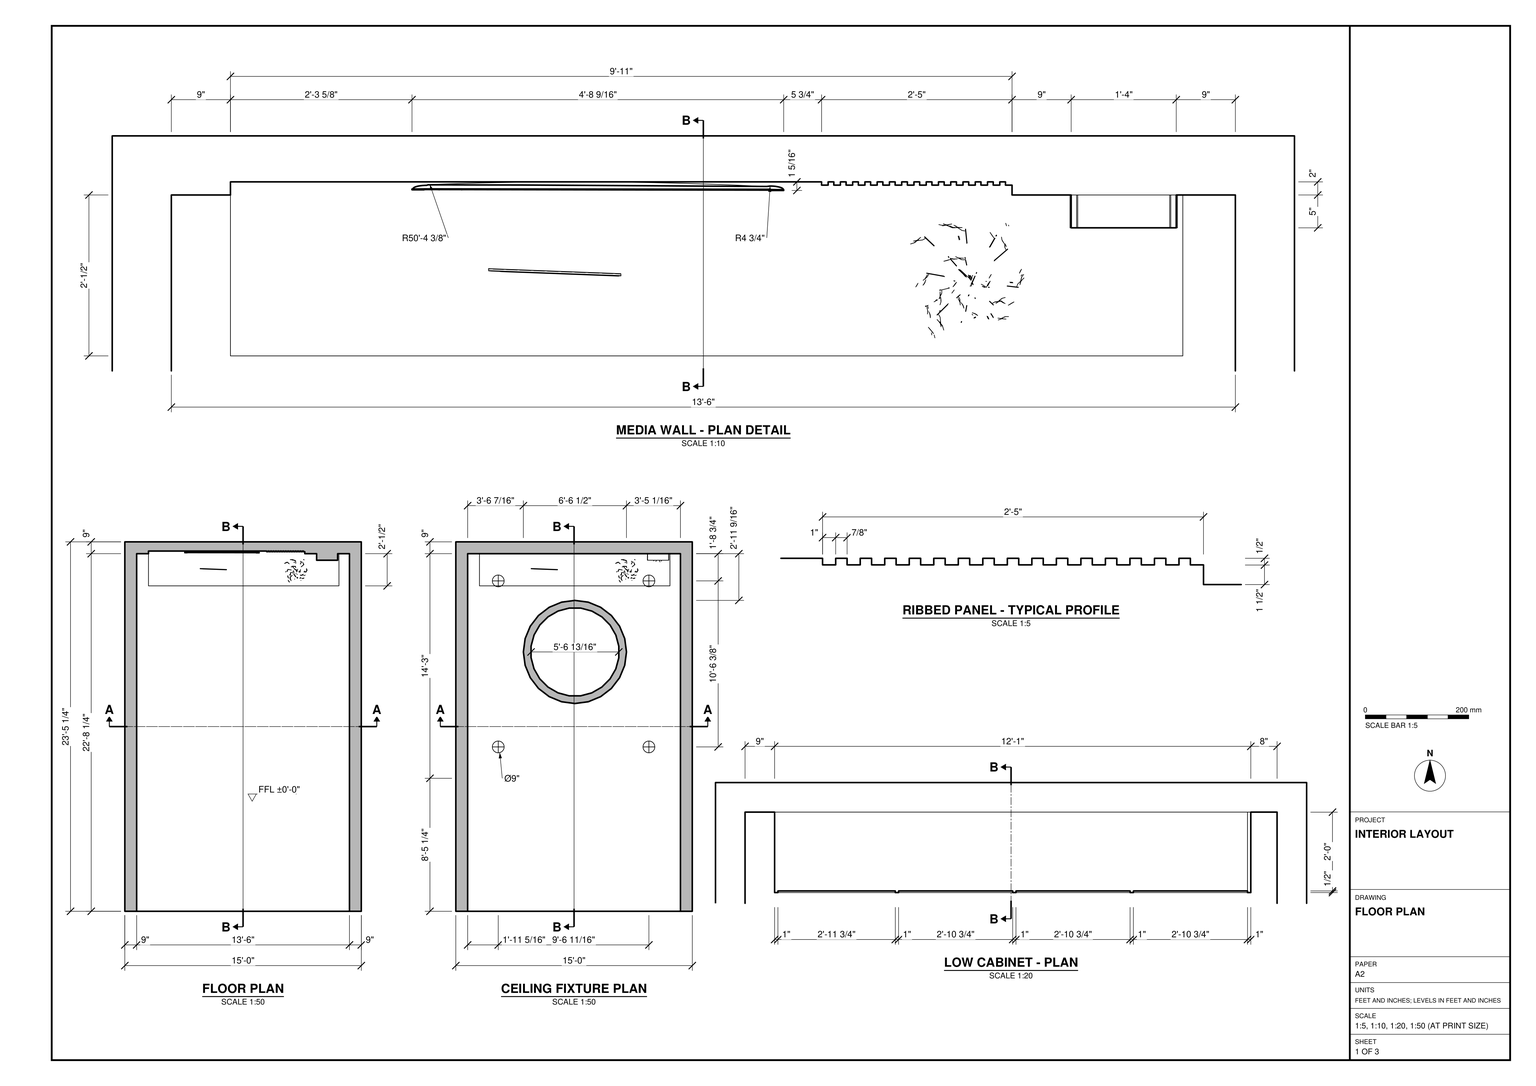
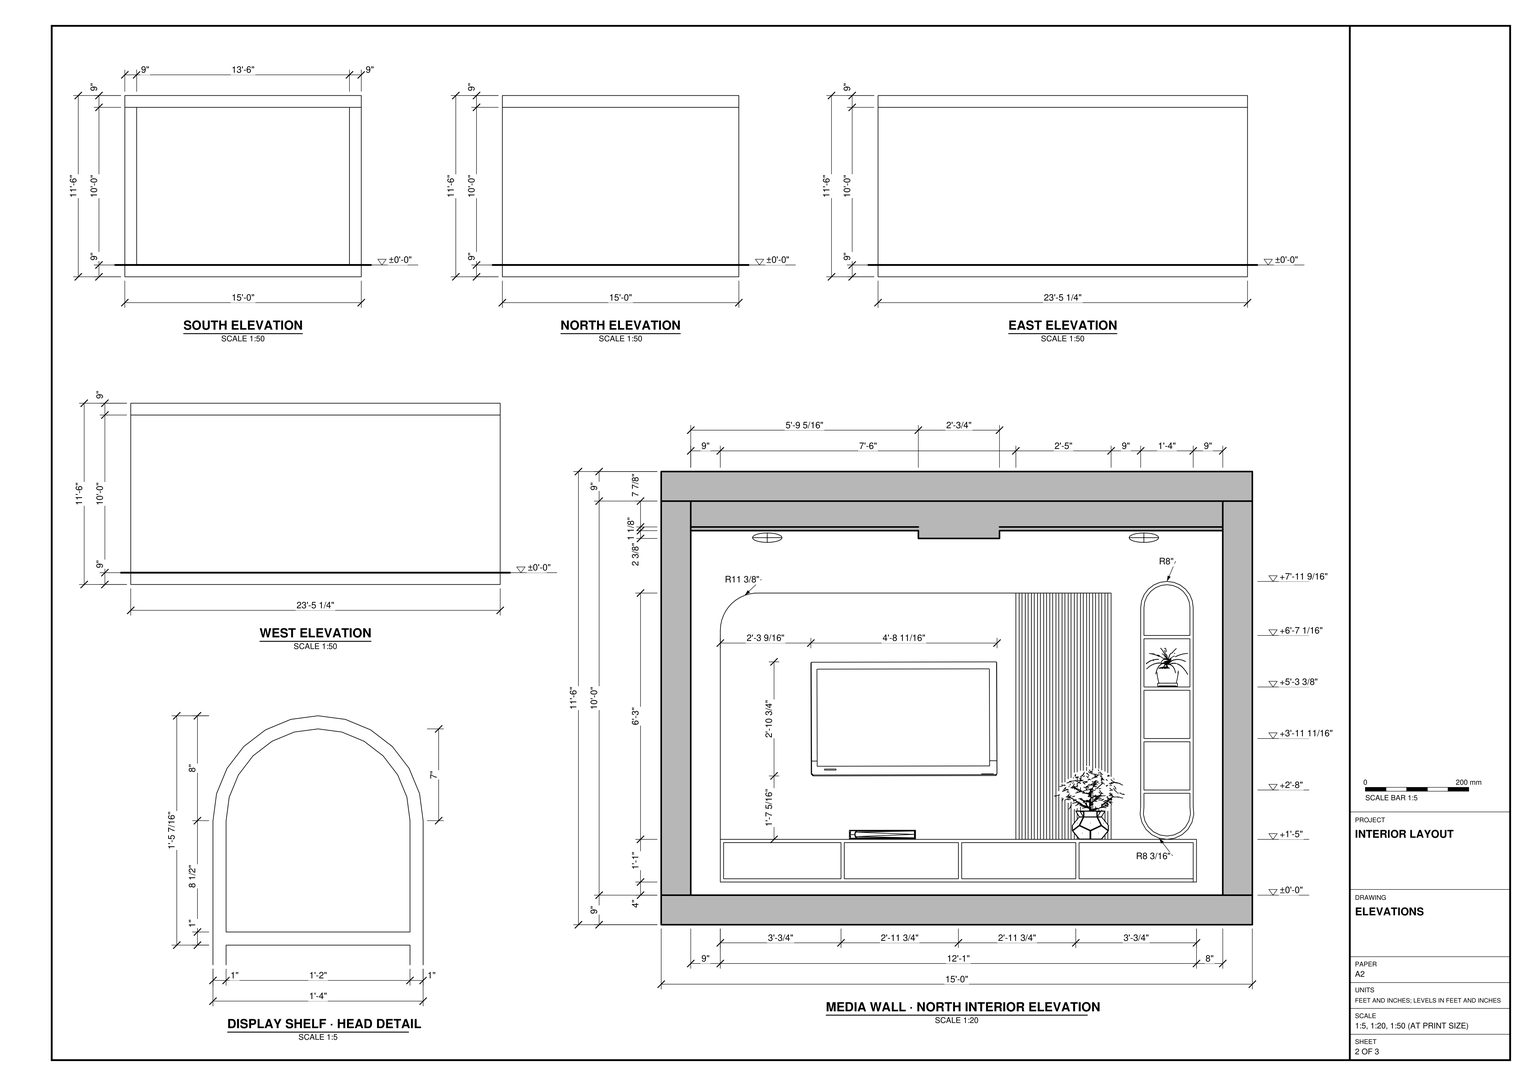
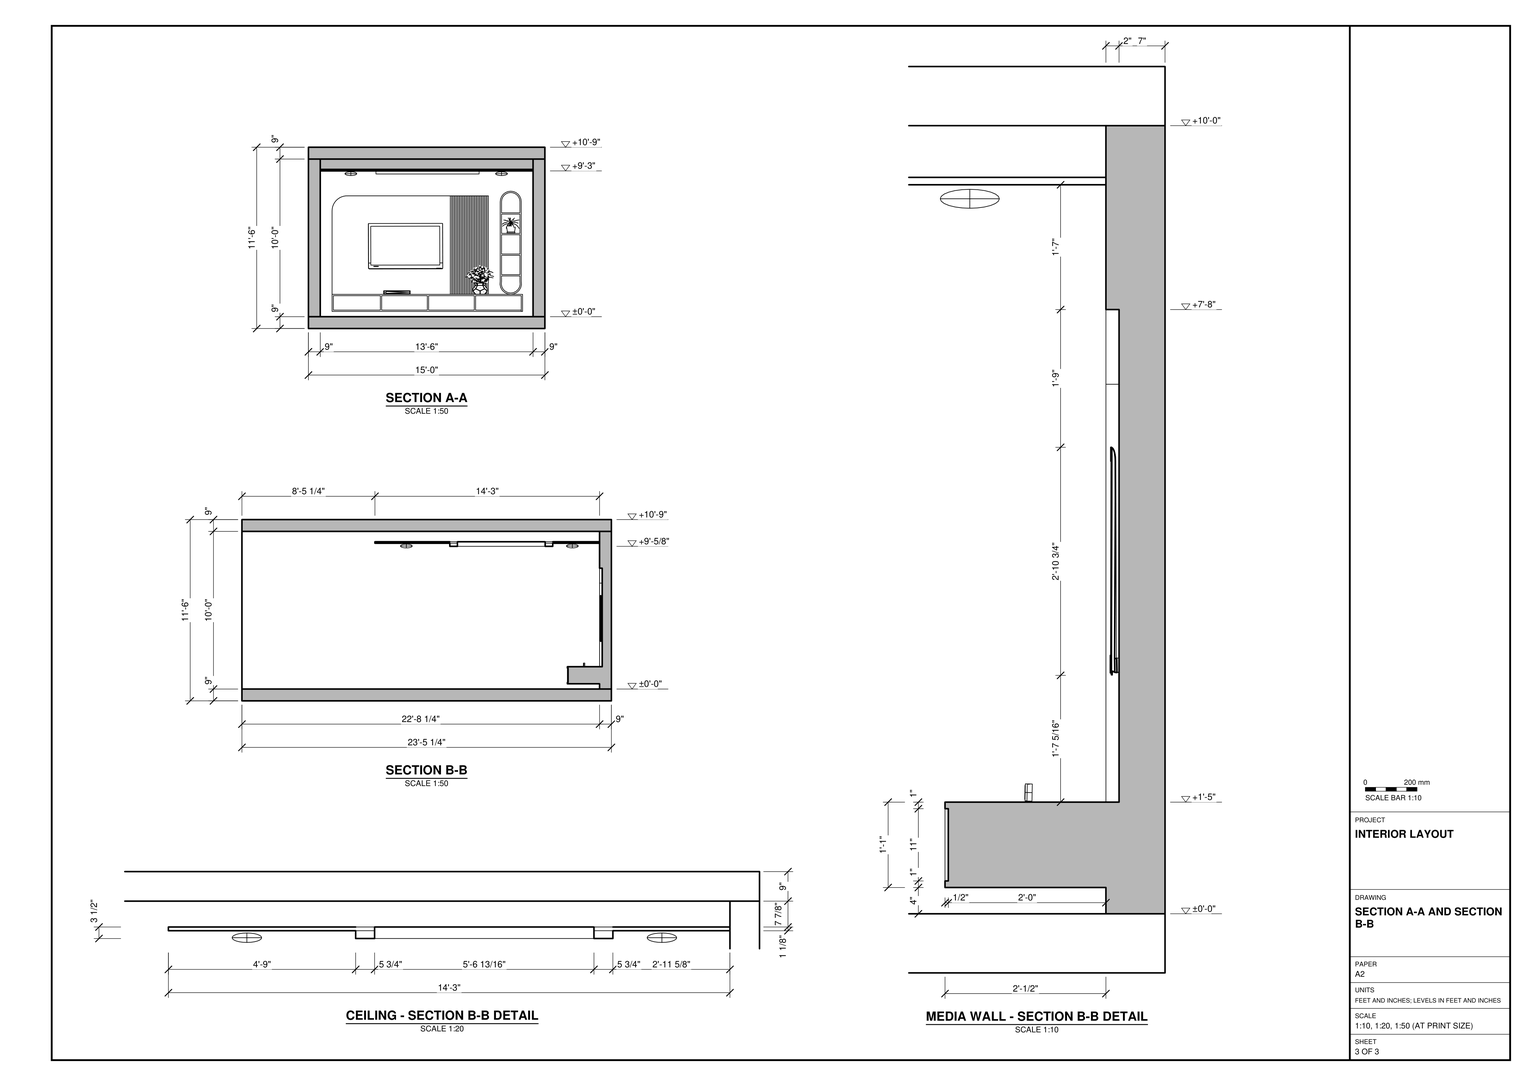
Build the media room in SketchUp from task_files/diagram_01.pdf. Work in feet and inches. Set the finished floor at ±0'-0" and make the shell 15'-0" wide, 23'-5 1/4" long and 11'-6" high overall. Model the north wall and both side walls at 9" thick, leaving the south end open as shown in plan. Use 9" floor and roof slabs with 10'-0" clear between them.

Use the north interior elevation to lay out the media wall. Float the low cabinet above the floor and divide its front into four bays. Mount the television on the smooth panel with the rounded upper left corner. Form the vertical ribs to its right using the profile detail, then add the narrow open display shelf with rounded ends. Place the small media device and potted plants where shown. Use the ceiling plan and section B-B to position the lowered ceiling panel, central ring fixture and smaller ceiling lights.

Decor and loose items may be any suitable library components. Keep the walls, slabs, ceiling panel and each furniture or joinery piece in separate groups or components, and use components for repeated parts. Save one SketchUp model as output_files/media_room_with_built_in_cabinetry_and_ceiling_fixtures.skp.

# SketchUp Ruby script. Lengths in inches.
U = 1.inch
M = Sketchup.active_model
def pt(a) = Geom::Point3d.new(a.map { |v| v * U })
def face(e, loops, mat)
  f = e.add_face(loops[0].map { |a| pt(a) })
  loops[1..].each { |l| e.add_face(l.map { |a| pt(a) }).erase! }
  f.material = f.back_material = mat if mat
  f
end
# faces: each face lists its corners as indices into pts; further lists are holes
def faces(e, pts, list, mat = nil) = list.each { |f| face(e, (f[0].is_a?(Array) ? f : [f]).map { |l| l.map { |i| pts[i] } }, mat) }
# xy, xz, yz: faces in a plane at the given z, y or x. An outline is a flat list of corners, or four numbers for a rectangle; further outlines are holes
def ring(l) = l.size == 4 ? [[l[0], l[1]], [l[2], l[1]], [l[2], l[3]], [l[0], l[3]]] : l.each_slice(2).to_a
def flat(e, list, mat, &to3) = list.each { |f| face(e, (f[0].is_a?(Array) ? f : [f]).map { |l| ring(l).map { |u, v| to3.(u, v) } }, mat) }
def xy(e, z, list, mat = nil) = flat(e, list, mat) { |x, y| [x, y, z] }
def xz(e, y, list, mat = nil) = flat(e, list, mat) { |x, z| [x, y, z] }
def yz(e, x, list, mat = nil) = flat(e, list, mat) { |y, z| [x, y, z] }
def lines(e, pts, list) = list.each { |a, b| e.add_line(pt(pts[a]), pt(pts[b])) }
# prism: a flat outline (further loops are holes) pulled along v
def prism(e, loops, v, mat = nil)
  f = face(e, loops, mat); d = Geom::Vector3d.new(v.map { |x| x * U })
  f.pushpull(f.normal.samedirection?(d) ? d.length : -d.length)
end
def box(e, o, s, mat = nil) = prism(e, [[o, [o[0] + s[0], o[1], o[2]], [o[0] + s[0], o[1] + s[1], o[2]], [o[0], o[1] + s[1], o[2]]]], [0, 0, s[2]], mat)
def at(x, y, z, deg = 0) = Geom::Transformation.translation(pt([x, y, z])) * Geom::Transformation.rotation(ORIGIN, Z_AXIS, deg.degrees)
def axes(o, x, y, z) = Geom::Transformation.new([*x, 0, *y, 0, *z, 0, *pt(o).to_a, 1])
def part(name) = M.definitions.add(name)
# library, detail: a bought-in or finely detailed component or shape, given as its bounding box
def library(name, o, s) = part(name).tap { |d| box(d.entities, o, s) }
def detail(e, o, s) = box(e.add_group.entities, o, s)
def put(e, d, t, mat = nil) = e.add_instance(d, t).tap { |i| i.material = mat if mat }
def group(e, t, mat = nil) = e.add_group.tap { |g| g.transformation = t; g.material = mat if mat }.entities
root = M.entities
M.materials.add("Emissive").color = [239, 214, 214]
M.materials.add("[0014_DarkSalmon]").color = [235, 180, 161]
M.materials.add("[0024_OrangeRed]").color = [254, 124, 76]
M.materials.add("[0134_DimGray]").color = [105, 105, 105]
M.materials.add("[0136_Charcoal]").color = [35, 35, 35]
M.materials.add("[0137_Black]").color = [0, 0, 0]
M.materials.add("[Carrera Marble]").color = [207, 207, 207]
c1 = library("Flat panel television",[-0.83,-0.0625,-0.19],[1.35,37.19,23.93])
c2 = part("skpA6C3")
xy(c2.entities,2.36,[[-169.4375,74.49,-169.56,74.75,-167.28,75.78,-167.16,75.52]])
xy(c2.entities,2.39,[[-169.39,74.48,-167.18,75.48,-169.18,74.58],[-169.39,74.48,-167.1875,75.5,-169.39,74.5],[-169.39,74.48,-169.18,74.58,-167.1875,75.5],[-169.18,74.58,-167.18,75.48,-167.1875,75.5]])
xy(c2.entities,2.8,[[-169.39,74.49,-169.39,74.5,-167.1875,75.5,-167.18,75.49,-169.18,74.58]])
xy(c2.entities,2.83,[[-169.4375,74.49,-167.16,75.52,-167.28,75.78,-169.56,74.75]])
xz(c2.entities,74.49,[[-169.4375,2.59,-169.39,2.8,-169.4375,2.83]])
yz(c2.entities,-169.39,[[74.48,2.39,74.5,2.39,74.48,2.6],[74.5,2.39,74.5,2.6,74.48,2.6],[74.48,2.6,74.5,2.6,74.5,2.8],[74.48,2.6,74.5,2.8,74.49,2.8]])
yz(c2.entities,-167.18,[[75.48,2.39,75.44,2.6,75.4375,2.41],[75.48,2.39,75.49,2.6,75.44,2.79,75.44,2.6],[75.49,2.6,75.49,2.8,75.44,2.79]])
p = [[-167.18,75.48,2.39],[-169.39,74.48,2.39],[-167.16,75.52,2.36],[-169.4375,74.49,2.36],[-167.1875,75.5,2.39],[-167.1875,75.5,2.6],
  [-167.1875,75.5,2.8],[-169.39,74.5,2.8],[-169.39,74.5,2.6],[-169.39,74.5,2.39],[-169.4375,74.49,2.59],[-169.39,74.48,2.6],
  [-169.18,74.58,2.39],[-167.18,75.4375,2.41],[-169.15,74.55,2.41],[-167.18,75.44,2.6],[-169.19,74.52,2.48],[-169.23,74.56,2.46],
  [-169.56,74.75,2.36],[-169.56,74.75,2.59],[-167.28,75.78,2.59],[-167.28,75.78,2.36],[-167.16,75.52,2.59],[-167.18,75.49,2.6],
  [-169.22,74.52,2.6],[-169.25,74.55,2.6],[-169.19,74.53,2.73],[-169.39,74.49,2.8],[-169.23,74.56,2.73],[-167.18,75.44,2.79],
  [-169.56,74.75,2.83],[-167.28,75.78,2.83],[-167.16,75.52,2.83],[-167.18,75.49,2.8],[-169.15,74.55,2.79],[-169.18,74.58,2.8],
  [-169.4375,74.49,2.83]]
faces(c2.entities,p,[[0,1,2],[1,3,2],[4,5,6,7,8,9],[10,3,1],[11,10,1],[12,0,13,14],[15,16,13],[16,14,13],
  [17,12,14],[16,17,14],[18,19,20,21],[2,21,20,22],[22,23,0],[22,0,2],[4,0,23],[5,4,23],
  [24,25,16],[25,17,16],[16,15,26,24],[27,10,11],[28,25,24],[29,26,15],[28,24,26],[19,30,31,20],
  [22,20,31,32],[22,33,23],[32,33,22],[5,23,33],[6,5,33],[29,34,26],[35,28,26],[35,26,34],
  [32,36,33],[27,35,33,36],[35,34,29,33]])
c3 = part("speaker")
put(c3.entities,c2,axes([-348.49,31.79,126.79],[0,-0.40035,0.91636],[0,0.91636,0.40035],[-1,0,0]))
c4 = library("4",[-16.3,-15.81,0],[32.6,31.62,37.8])
c5 = library("granite type garden pot + desert rose wine plant",[-22.7,-22.54,0],[44.26,46.62,61.81])
c6 = part("Group35\#1")
p = [[0,0,0],[0,0,-0.26],[-0.06,0,-0.26],[0.39,-0.44,0],[-0.39,-0.44,0],[0.39,0.44,0],
  [0.39,0,0],[-0.39,0.44,0],[0.06,0,-0.26],[-0.39,0,0],[0,0,-0.42]]
lines(c6.entities,p,[[0,1],[1,2],[3,4],[5,6],[7,5],[1,8],[9,0],[0,6],[8,10],[4,9],[6,3],[2,10],
  [9,7]])
c7 = part("Rectangle Light")
put(c7.entities,c6,at(0,0,0))
c8 = library("Sphere Light",[-4.5,-4.5,-4.5],[9,9,9])
xy(root,-9,[[0,0,180,281.25]])
xy(root,0,[[0,0,9,0,9,272.25,171,272.25,171,0,180,0,180,281.25,0,281.25],[9,0,171,272.25]])
xy(root,4,[[18,247.75,162,272.25],[162,247.75,163,272.25]])
xy(root,5,[[19,247.75,54.75,248.25],[55.75,247.75,90.5,248.25],[91.5,247.75,126.25,248.25],[127.25,247.75,162,248.25]])
xy(root,16,[[19,247.75,54.75,248.25],[55.75,247.75,90.5,248.25],[91.5,247.75,126.25,248.25],[127.25,247.75,162,248.25]])
xy(root,17,[[18,247.75,163,247.75,163,272.25,137,272.25,137,273.75,136,273.75,136,274.25,135.13,274.25,135.13,273.75,134.13,273.75,134.13,274.25,133.27,274.25,133.27,273.75,132.27,273.75,132.27,274.25,131.4,274.25,131.4,273.75,130.4,273.75,130.4,274.25,129.53,274.25,129.53,273.75,128.53,273.75,128.53,274.25,127.67,274.25,127.67,273.75,126.67,273.75,126.67,274.25,125.8,274.25,125.8,273.75,124.8,273.75,124.8,274.25,123.93,274.25,123.93,273.75,122.93,273.75,122.93,274.25,122.07,274.25,122.07,273.75,121.07,273.75,121.07,274.25,120.2,274.25,120.2,273.75,119.2,273.75,119.2,274.25,118.33,274.25,118.33,273.75,117.33,273.75,117.33,274.25,116.47,274.25,116.47,273.75,115.47,273.75,115.47,274.25,114.6,274.25,114.6,273.75,113.6,273.75,113.6,274.25,112.73,274.25,112.73,273.75,111.73,273.75,111.73,274.25,110.87,274.25,110.87,273.75,109.87,273.75,109.87,274.25,109,274.25,109,273.75,108,273.75,108,274.25,18,274.25]],"[Carrera Marble]")
xy(root,31.02,[[147,267.25,161,272.25]])
xy(root,32.02,[[147,267.25,161,272.25]],"[0134_DimGray]")
xy(root,46.71,[[147,267.25,161,272.25]])
xy(root,47.71,[[147,267.25,161,272.25]],"[0134_DimGray]")
xy(root,62.39,[[147,267.25,161,272.25]])
xy(root,63.39,[[147,267.25,161,272.25]])
xy(root,78.08,[[147,267.25,161,272.25]])
xy(root,79.08,[[147,267.25,161,272.25]])
xy(root,92,[[30,272.25,30,274.25,108,274.25,108,273.75,109,273.75,109,274.25,109.87,274.25,109.87,273.75,110.87,273.75,110.87,274.25,111.73,274.25,111.73,273.75,112.73,273.75,112.73,274.25,113.6,274.25,113.6,273.75,114.6,273.75,114.6,274.25,115.47,274.25,115.47,273.75,116.47,273.75,116.47,274.25,117.33,274.25,117.33,273.75,118.33,273.75,118.33,274.25,119.2,274.25,119.2,273.75,120.2,273.75,120.2,274.25,121.07,274.25,121.07,273.75,122.07,273.75,122.07,274.25,122.93,274.25,122.93,273.75,123.93,273.75,123.93,274.25,124.8,274.25,124.8,273.75,125.8,273.75,125.8,274.25,126.67,274.25,126.67,273.75,127.67,273.75,127.67,274.25,128.53,274.25,128.53,273.75,129.53,273.75,129.53,274.25,130.4,274.25,130.4,273.75,131.4,273.75,131.4,274.25,132.27,274.25,132.27,273.75,133.27,273.75,133.27,274.25,134.13,274.25,134.13,273.75,135.13,273.75,135.13,274.25,136,274.25,136,273.75,137,273.75,137,272.25]],"Emissive")
xy(root,120,[[0,0,0,281.25,180,281.25,180,0,171,0,171,272.25,9,272.25,9,0]])
xy(root,120,[[9,0,171,272.25]],"[0014_DarkSalmon]")
xy(root,129,[[0,0,180,281.25]])
xz(root,0,[[0,-9,180,0],[0,0,9,120],[9,0,171,120],[171,0,180,120],[0,120,180,129]])
xz(root,247.75,[[[18,4,162,4,162,5,127.25,5,127.25,16,162,16,162,4,163,4,163,17,18,17],[19,5,54.75,16],[91.5,5,126.25,16],[55.75,5,90.5,16]]],"[0136_Charcoal]")
xz(root,248.25,[[19,5,54.75,16],[55.75,5,90.5,16],[91.5,5,126.25,16],[127.25,5,162,16]],"[Carrera Marble]")
xz(root,267.25,[[[154,17,156.41,17.36,158.61,18.42,160.4,20.08,161.625,22.1875,162.18,24.57,162,27,162,87.54,161.73,89.62,160.93,91.54,159.66,93.2,158,94.47,156.07,95.27,154,95.54,151.93,95.27,150,94.47,148.34,93.2,147.07,91.54,146.27,89.62,146,87.54,146,27,145.82,24.57,146.375,22.1875,147.6,20.08,149.39,18.42,151.59,17.36],[147,63.39,161,78.08],[147,47.71,161,62.39],[147,32.02,161,46.71],[147,79.08,147,87.54,147.24,89.36,147.9375,91.04,149.05,92.49,150.5,93.61,152.1875,94.31,154,94.54,155.8125,94.31,157.5,93.61,158.95,92.49,160.0625,91.04,160.76,89.36,161,87.54,161,79.08],[154,18.01,151.88,18.33,149.96,19.26,148.39,20.71,147.3125,22.56,146.83,24.64,147,26.96,147,31.02,161,31.02,161,26.96,161.17,24.64,160.6875,22.56,159.61,20.71,158.04,19.26,156.12,18.33]]],"[0137_Black]")
xz(root,272.25,[[[9,0,171,120],[18,4,18,80.625,18.1,82.16,18.41,83.67,18.93,85.125,19.63,86.5,20.51,87.76,21.55,88.89,22.74,89.875,24.05,90.6875,25.46,91.32,26.9375,91.75,28.46,91.98,30,92,137,92,137,17,163,17,163,4],[154,17,151.59,17.36,149.39,18.42,147.6,20.08,146.375,22.1875,145.82,24.57,146,27,146,87.54,146.27,89.62,147.07,91.54,148.34,93.2,150,94.47,151.93,95.27,154,95.54,156.07,95.27,158,94.47,159.66,93.2,160.93,91.54,161.73,89.62,162,87.54,162,27,162.18,24.57,161.625,22.1875,160.4,20.08,158.61,18.42,156.41,17.36]]],"[0014_DarkSalmon]")
xz(root,272.25,[[154,18.01,156.12,18.33,158.04,19.26,159.61,20.71,160.6875,22.56,161.17,24.64,161,26.96,161,31.02,147,31.02,147,26.96,146.83,24.64,147.3125,22.56,148.39,20.71,149.96,19.26,151.88,18.33],[147,32.02,161,46.71],[147,47.71,161,62.39],[147,63.39,161,78.08],[147,79.08,161,79.08,161,87.54,160.76,89.36,160.0625,91.04,158.95,92.49,157.5,93.61,155.8125,94.31,154,94.54,152.1875,94.31,150.5,93.61,149.05,92.49,147.9375,91.04,147.24,89.36,147,87.54]],"[0134_DimGray]")
xz(root,273.75,[[130.4,17,131.4,92],[132.27,17,133.27,92],[134.13,17,135.13,92],[136,17,137,92]])
xz(root,273.75,[[108,17,109,92],[109.87,17,110.87,92],[111.73,17,112.73,92],[113.6,17,114.6,92],[115.47,17,116.47,92],
  [117.33,17,118.33,92],[119.2,17,120.2,92],[121.07,17,122.07,92],[122.93,17,123.93,92],[124.8,17,125.8,92],
  [126.67,17,127.67,92],[128.53,17,129.53,92]],"[0024_OrangeRed]")
xz(root,274.25,[[109,17,109.87,92],[110.87,17,111.73,92],[112.73,17,113.6,92],[114.6,17,115.47,92],[116.47,17,117.33,92],
  [118.33,17,119.2,92],[120.2,17,121.07,92],[122.07,17,122.93,92],[123.93,17,124.8,92],[125.8,17,126.67,92],
  [127.67,17,128.53,92],[129.53,17,130.4,92]])
xz(root,274.25,[[131.4,17,132.27,92],[133.27,17,134.13,92],[135.13,17,136,92]],"[0024_OrangeRed]")
xz(root,274.25,[[18,17,108,17,108,92,30,92,28.46,91.98,26.9375,91.75,25.46,91.32,24.05,90.6875,22.74,89.875,21.55,88.89,20.51,87.76,19.63,86.5,18.93,85.125,18.41,83.67,18.1,82.16,18,80.625]],"[Carrera Marble]")
xz(root,281.25,[[0,-9,180,0],[0,0,180,120],[0,120,180,129]])
yz(root,0,[[0,-9,281.25,0],[0,0,281.25,120],[0,120,281.25,129]])
yz(root,9,[[0,0,272.25,120]],"[0014_DarkSalmon]")
yz(root,18,[[247.75,4,272.25,5],[247.75,5,272.25,16],[247.75,16,272.25,17]])
yz(root,18,[[272.25,17,274.25,80.625]],"Emissive")
yz(root,19,[[247.75,5,248.25,16]])
yz(root,54.75,[[247.75,5,248.25,16]])
yz(root,55.75,[[247.75,5,248.25,16]])
yz(root,90.5,[[247.75,5,248.25,16]])
yz(root,91.5,[[247.75,5,248.25,16]])
yz(root,108,[[273.75,17,274.25,92]])
yz(root,109,[[273.75,17,274.25,92]])
yz(root,109.87,[[273.75,17,274.25,92]])
yz(root,110.87,[[273.75,17,274.25,92]])
yz(root,111.73,[[273.75,17,274.25,92]])
yz(root,112.73,[[273.75,17,274.25,92]])
yz(root,113.6,[[273.75,17,274.25,92]])
yz(root,114.6,[[273.75,17,274.25,92]])
yz(root,115.47,[[273.75,17,274.25,92]])
yz(root,116.47,[[273.75,17,274.25,92]])
yz(root,117.33,[[273.75,17,274.25,92]])
yz(root,118.33,[[273.75,17,274.25,92]])
yz(root,119.2,[[273.75,17,274.25,92]])
yz(root,120.2,[[273.75,17,274.25,92]])
yz(root,121.07,[[273.75,17,274.25,92]])
yz(root,122.07,[[273.75,17,274.25,92]])
yz(root,122.93,[[273.75,17,274.25,92]])
yz(root,123.93,[[273.75,17,274.25,92]])
yz(root,124.8,[[273.75,17,274.25,92]])
yz(root,125.8,[[273.75,17,274.25,92]])
yz(root,126.25,[[247.75,5,248.25,16]])
yz(root,126.67,[[273.75,17,274.25,92]])
yz(root,127.25,[[247.75,5,248.25,16]])
yz(root,127.67,[[273.75,17,274.25,92]])
yz(root,128.53,[[273.75,17,274.25,92]])
yz(root,129.53,[[273.75,17,274.25,92]])
yz(root,130.4,[[273.75,17,274.25,92]])
yz(root,131.4,[[273.75,17,274.25,92]])
yz(root,132.27,[[273.75,17,274.25,92]])
yz(root,133.27,[[273.75,17,274.25,92]])
yz(root,134.13,[[273.75,17,274.25,92]])
yz(root,135.13,[[273.75,17,274.25,92]])
yz(root,136,[[273.75,17,274.25,92]])
yz(root,137,[[272.25,17,273.75,92]],"Emissive")
yz(root,146,[[267.25,27,272.25,87.54]],"[0134_DimGray]")
yz(root,147,[[267.25,26.96,272.25,31.02]])
yz(root,147,[[267.25,32.02,272.25,46.71],[267.25,47.71,272.25,62.39],[267.25,63.39,272.25,78.08],[267.25,79.08,272.25,87.54]],"[0134_DimGray]")
yz(root,161,[[267.25,63.39,272.25,78.08]])
yz(root,161,[[267.25,26.96,272.25,31.02],[267.25,32.02,272.25,46.71],[267.25,47.71,272.25,62.39],[267.25,79.08,272.25,87.54]],"[0134_DimGray]")
yz(root,162,[[247.75,4,248.25,5],[247.75,5,248.25,16],[267.25,27,272.25,87.54]])
yz(root,163,[[247.75,4,272.25,17]])
yz(root,171,[[0,0,272.25,120]],"[0014_DarkSalmon]")
yz(root,180,[[0,-9,281.25,0],[0,0,281.25,120],[0,120,281.25,129]])
p = [[151.59,272.25,17.36],[154,272.25,17],[154,267.25,17],[151.59,267.25,17.36],[156.41,272.25,17.36],[156.41,267.25,17.36],
  [149.39,272.25,18.42],[149.39,267.25,18.42],[158.61,272.25,18.42],[158.61,267.25,18.42],[154,272.25,18.01],[151.88,272.25,18.33],
  [151.88,267.25,18.33],[154,267.25,18.01],[156.12,272.25,18.33],[156.12,267.25,18.33],[149.96,272.25,19.26],[149.96,267.25,19.26],
  [158.04,272.25,19.26],[158.04,267.25,19.26],[147.6,272.25,20.08],[147.6,267.25,20.08],[160.4,272.25,20.08],[160.4,267.25,20.08],
  [148.39,272.25,20.71],[148.39,267.25,20.71],[159.61,272.25,20.71],[159.61,267.25,20.71],[146.375,272.25,22.1875],[146.375,267.25,22.1875],
  [161.625,272.25,22.1875],[161.625,267.25,22.1875],[147.3125,272.25,22.56],[147.3125,267.25,22.56],[160.6875,272.25,22.56],[160.6875,267.25,22.56],
  [145.82,272.25,24.57],[145.82,267.25,24.57],[162.18,272.25,24.57],[162.18,267.25,24.57],[146.83,272.25,24.64],[146.83,267.25,24.64],
  [161.17,272.25,24.64],[161.17,267.25,24.64],[146,272.25,27],[146,267.25,27],[147,272.25,26.96],[147,267.25,26.96],
  [161,272.25,26.96],[161,267.25,26.96],[162,272.25,27],[162,267.25,27],[18.1,272.25,82.16],[18,272.25,80.625],
  [18,274.25,80.625],[18.1,274.25,82.16],[18.41,272.25,83.67],[18.41,274.25,83.67],[18.93,272.25,85.125],[18.93,274.25,85.125],
  [19.63,272.25,86.5],[19.63,274.25,86.5],[20.51,272.25,87.76],[20.51,274.25,87.76],[146.27,272.25,89.62],[146,272.25,87.54],
  [146,267.25,87.54],[146.27,267.25,89.62],[147,272.25,87.54],[147.24,272.25,89.36],[147.24,267.25,89.36],[147,267.25,87.54],
  [160.76,272.25,89.36],[161,272.25,87.54],[161,267.25,87.54],[160.76,267.25,89.36],[162,272.25,87.54],[161.73,272.25,89.62],
  [161.73,267.25,89.62],[162,267.25,87.54],[21.55,272.25,88.89],[21.55,274.25,88.89],[22.74,272.25,89.875],[22.74,274.25,89.875],
  [147.9375,272.25,91.04],[147.9375,267.25,91.04],[160.0625,272.25,91.04],[160.0625,267.25,91.04],[147.07,272.25,91.54],[147.07,267.25,91.54],
  [160.93,272.25,91.54],[160.93,267.25,91.54],[24.05,272.25,90.6875],[24.05,274.25,90.6875],[25.46,272.25,91.32],[25.46,274.25,91.32],
  [149.05,272.25,92.49],[149.05,267.25,92.49],[158.95,272.25,92.49],[158.95,267.25,92.49],[26.9375,272.25,91.75],[26.9375,274.25,91.75],
  [148.34,272.25,93.2],[148.34,267.25,93.2],[159.66,272.25,93.2],[159.66,267.25,93.2],[28.46,272.25,91.98],[28.46,274.25,91.98],
  [30,272.25,92],[30,274.25,92],[150.5,272.25,93.61],[150.5,267.25,93.61],[157.5,272.25,93.61],[157.5,267.25,93.61],
  [150,272.25,94.47],[150,267.25,94.47],[158,272.25,94.47],[158,267.25,94.47],[152.1875,272.25,94.31],[152.1875,267.25,94.31],
  [155.8125,272.25,94.31],[155.8125,267.25,94.31],[154,272.25,94.54],[154,267.25,94.54],[151.93,272.25,95.27],[151.93,267.25,95.27],
  [156.07,272.25,95.27],[156.07,267.25,95.27],[154,272.25,95.54],[154,267.25,95.54]]
faces(root,p,[[0,1,2,3],[1,4,5,2],[6,0,3,7],[4,8,9,5],[20,6,7,21],[8,22,23,9],[28,20,21,29],[22,30,31,23],
  [36,28,29,37],[30,38,39,31],[44,36,37,45],[38,50,51,39],[64,65,66,67],[76,77,78,79],[88,64,67,89],[77,90,91,78],
  [102,88,89,103],[90,104,105,91],[114,102,103,115],[104,116,117,105],[124,114,115,125],[116,126,127,117],[128,124,125,129],[126,128,129,127]])
faces(root,p,[[10,11,12,13],[14,10,13,15],[11,16,17,12],[18,14,15,19],[16,24,25,17],[26,18,19,27],[24,32,33,25],[34,26,27,35],
  [32,40,41,33],[42,34,35,43],[40,46,47,41],[48,42,43,49],[68,69,70,71],[72,73,74,75],[69,84,85,70],[86,72,75,87],
  [84,96,97,85],[98,86,87,99],[96,110,111,97],[112,98,99,113],[110,118,119,111],[120,112,113,121],[118,122,123,119],[122,120,121,123]],"[0134_DimGray]")
faces(root,p,[[52,53,54,55],[56,52,55,57],[58,56,57,59],[60,58,59,61],[62,60,61,63],[80,62,63,81],[82,80,81,83],[92,82,83,93],
  [94,92,93,95],[100,94,95,101],[106,100,101,107],[108,106,107,109]],"Emissive")
put(root,c1,axes([45.67,273.42,36.58],[0,-1,0],[1.524,0,0],[0,0,1.452]),"Emissive")
put(root,c3,axes([40.02,58.69,-1922.88],[0.00065,-0.09897,-5.53808],[0.0396,0.99906,-0.01785],[8.07018,-0.31978,0.00667]))
put(root,c4,axes([154.11,269.94,63.39],[0.39618,0,0],[0,0.25276,0],[0,0,0.31624]))
put(root,c5,axes([130.6875,259.11,17],[0.50622,0,0],[0,0.504,0],[0,0,0.37]))
put(root,c7,axes([90.5,272.24,3.56],[-184.66732,0,0],[0,0,-1],[0,1,0]))
g1 = group(root,at(9,101.25,107.43))
xy(g1,1.2,[[[81.66,56.9375,71.5,58.28,62.04,62.2,53.91,68.43,47.67,76.5625,43.75,86.03,42.41,96.1875,43.75,106.35,47.67,115.8125,53.91,123.94,62.04,130.18,71.5,134.1,81.66,135.4375,91.82,134.1,101.29,130.18,109.42,123.94,115.65,115.8125,119.58,106.35,120.91,96.1875,119.58,86.03,115.65,76.5625,109.42,68.43,101.29,62.2,91.82,58.28],[85.99,62.78,94.49,65.04,102.12,69.42,108.35,75.625,112.76,83.23,115.05,91.72,115.07,100.52,112.8125,109.02,108.43,116.64,102.23,122.87,94.62,127.28,86.13,129.58,77.33,129.6,68.84,127.34,61.21,122.96,54.98,116.75,50.57,109.14,48.27,100.65,48.25,91.86,50.51,83.36,54.89,75.74,61.1,69.5,68.71,65.09,77.2,62.8]]])
xy(g1,3.57,[[[0,0,162,171],[81.66,56.9375,91.82,58.28,101.29,62.2,109.42,68.43,115.65,76.5625,119.58,86.03,120.91,96.1875,119.58,106.35,115.65,115.8125,109.42,123.94,101.29,130.18,91.82,134.1,81.66,135.4375,71.5,134.1,62.04,130.18,53.91,123.94,47.67,115.8125,43.75,106.35,42.41,96.1875,43.75,86.03,47.67,76.5625,53.91,68.43,62.04,62.2,71.5,58.28]]])
xy(g1,4.7,[[[0,0,162,171],[81.66,56.9375,71.5,58.28,62.04,62.2,53.91,68.43,47.67,76.5625,43.75,86.03,42.41,96.1875,43.75,106.35,47.67,115.8125,53.91,123.94,62.04,130.18,71.5,134.1,81.66,135.4375,91.82,134.1,101.29,130.18,109.42,123.94,115.65,115.8125,119.58,106.35,120.91,96.1875,119.58,86.03,115.65,76.5625,109.42,68.43,101.29,62.2,91.82,58.28]],[85.99,62.78,77.2,62.8,68.71,65.09,61.1,69.5,54.89,75.74,50.51,83.36,48.25,91.86,48.27,100.65,50.57,109.14,54.98,116.75,61.21,122.96,68.84,127.34,77.33,129.6,86.13,129.58,94.62,127.28,102.23,122.87,108.43,116.64,112.8125,109.02,115.07,100.52,115.05,91.72,112.76,83.23,108.35,75.625,102.12,69.42,94.49,65.04]])
xz(g1,0,[[0,3.57,162,4.7]])
xz(g1,171,[[0,3.57,162,4.7]])
yz(g1,0,[[0,3.57,171,4.7]])
yz(g1,162,[[0,3.57,171,4.7]])
p = [[81.66,56.9375,1.2],[81.66,56.9375,3.57],[71.5,58.28,3.57],[71.5,58.28,1.2],[91.82,58.28,1.2],[91.82,58.28,3.57],
  [62.04,62.2,3.57],[62.04,62.2,1.2],[101.29,62.2,1.2],[101.29,62.2,3.57],[53.91,68.43,3.57],[53.91,68.43,1.2],
  [109.42,68.43,1.2],[109.42,68.43,3.57],[68.71,65.09,4.7],[77.2,62.8,4.7],[77.2,62.8,1.2],[68.71,65.09,1.2],
  [85.99,62.78,4.7],[85.99,62.78,1.2],[94.49,65.04,4.7],[94.49,65.04,1.2],[102.12,69.42,4.7],[102.12,69.42,1.2],
  [61.1,69.5,4.7],[61.1,69.5,1.2],[47.67,76.5625,3.57],[47.67,76.5625,1.2],[115.65,76.5625,1.2],[115.65,76.5625,3.57],
  [108.35,75.625,4.7],[108.35,75.625,1.2],[54.89,75.74,4.7],[54.89,75.74,1.2],[112.76,83.23,4.7],[112.76,83.23,1.2],
  [50.51,83.36,4.7],[50.51,83.36,1.2],[43.75,86.03,3.57],[43.75,86.03,1.2],[119.58,86.03,1.2],[119.58,86.03,3.57],
  [115.05,91.72,4.7],[115.05,91.72,1.2],[48.25,91.86,4.7],[48.25,91.86,1.2],[42.41,96.1875,3.57],[42.41,96.1875,1.2],
  [120.91,96.1875,1.2],[120.91,96.1875,3.57],[115.07,100.52,4.7],[115.07,100.52,1.2],[48.27,100.65,4.7],[48.27,100.65,1.2],
  [43.75,106.35,3.57],[43.75,106.35,1.2],[119.58,106.35,1.2],[119.58,106.35,3.57],[112.8125,109.02,4.7],[112.8125,109.02,1.2],
  [50.57,109.14,4.7],[50.57,109.14,1.2],[47.67,115.8125,3.57],[47.67,115.8125,1.2],[115.65,115.8125,1.2],[115.65,115.8125,3.57],
  [108.43,116.64,4.7],[108.43,116.64,1.2],[54.98,116.75,4.7],[54.98,116.75,1.2],[53.91,123.94,3.57],[53.91,123.94,1.2],
  [109.42,123.94,1.2],[109.42,123.94,3.57],[102.23,122.87,4.7],[102.23,122.87,1.2],[61.21,122.96,4.7],[61.21,122.96,1.2],
  [94.62,127.28,4.7],[94.62,127.28,1.2],[68.84,127.34,4.7],[68.84,127.34,1.2],[62.04,130.18,3.57],[62.04,130.18,1.2],
  [101.29,130.18,1.2],[101.29,130.18,3.57],[77.33,129.6,4.7],[77.33,129.6,1.2],[86.13,129.58,4.7],[86.13,129.58,1.2],
  [71.5,134.1,3.57],[71.5,134.1,1.2],[91.82,134.1,1.2],[91.82,134.1,3.57],[81.66,135.4375,3.57],[81.66,135.4375,1.2],
  [62.04,62.2,4.7],[115.65,76.5625,4.7],[119.58,106.35,4.7],[109.42,123.94,4.7],[53.91,68.43,4.7],[119.58,86.03,4.7],
  [101.29,130.18,4.7],[81.66,135.4375,4.7],[62.04,130.18,4.7],[43.75,106.35,4.7],[91.82,134.1,4.7],[42.41,96.1875,4.7],
  [109.42,68.43,4.7],[43.75,86.03,4.7],[71.5,58.28,4.7],[101.29,62.2,4.7],[53.91,123.94,4.7],[115.65,115.8125,4.7],
  [47.67,115.8125,4.7],[120.91,96.1875,4.7],[71.5,134.1,4.7],[47.67,76.5625,4.7],[81.66,56.9375,4.7],[91.82,58.28,4.7]]
faces(g1,p,[[0,1,2,3],[4,5,1,0],[3,2,6,7],[8,9,5,4],[7,6,10,11],[12,13,9,8],[14,15,16,17],[15,18,19,16],
  [18,20,21,19],[20,22,23,21],[24,14,17,25],[11,10,26,27],[28,29,13,12],[22,30,31,23],[32,24,25,33],[30,34,35,31],
  [36,32,33,37],[27,26,38,39],[40,41,29,28],[34,42,43,35],[44,36,37,45],[39,38,46,47],[48,49,41,40],[42,50,51,43],
  [52,44,45,53],[47,46,54,55],[56,57,49,48],[50,58,59,51],[60,52,53,61],[55,54,62,63],[64,65,57,56],[58,66,67,59],
  [68,60,61,69],[63,62,70,71],[72,73,65,64],[66,74,75,67],[76,68,69,77],[74,78,79,75],[80,76,77,81],[71,70,82,83],
  [84,85,73,72],[86,80,81,87],[78,88,89,79],[88,86,87,89],[83,82,90,91],[92,93,85,84],[91,90,94,95],[95,94,93,92]],"Emissive")
lines(g1,p,[[96,6],[97,29],[98,57],[99,73],[100,10],[101,41],[102,85],[103,94],[104,82],[105,54],[106,93],[107,46],
  [108,13],[109,38],[110,2],[111,9],[112,70],[113,65],[114,62],[115,49],[116,90],[117,26],[118,1],[119,5]])
put(g1,c8,axes([23.29,150.28,1.44],[1,0,0],[0,1,0],[0,0,0.32]))
put(g1,c8,axes([23.29,23.9,1.44],[1,0,0],[0,1,0],[0,0,0.32]))
put(g1,c8,axes([137.98,23.9,1.44],[1,0,0],[0,1,0],[0,0,0.32]))
put(g1,c8,axes([137.98,150.28,1.44],[1,0,0],[0,1,0],[0,0,0.32]))
